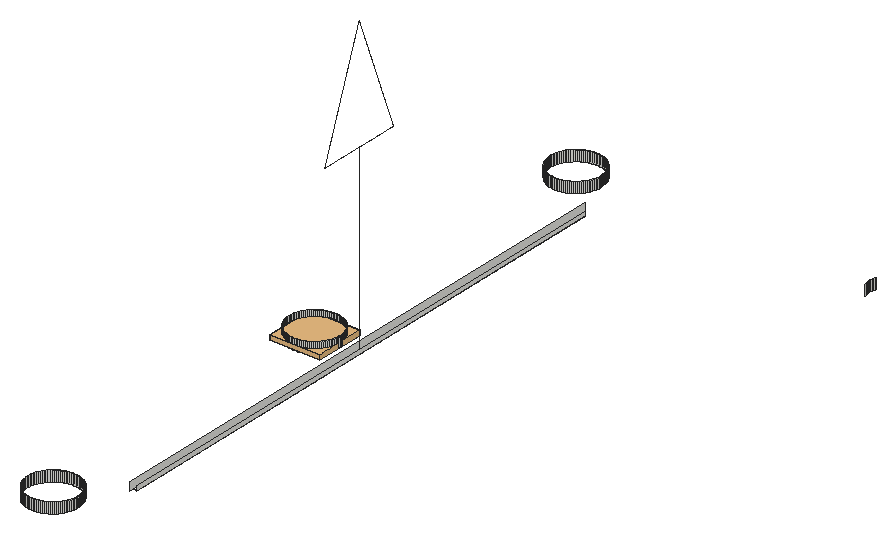
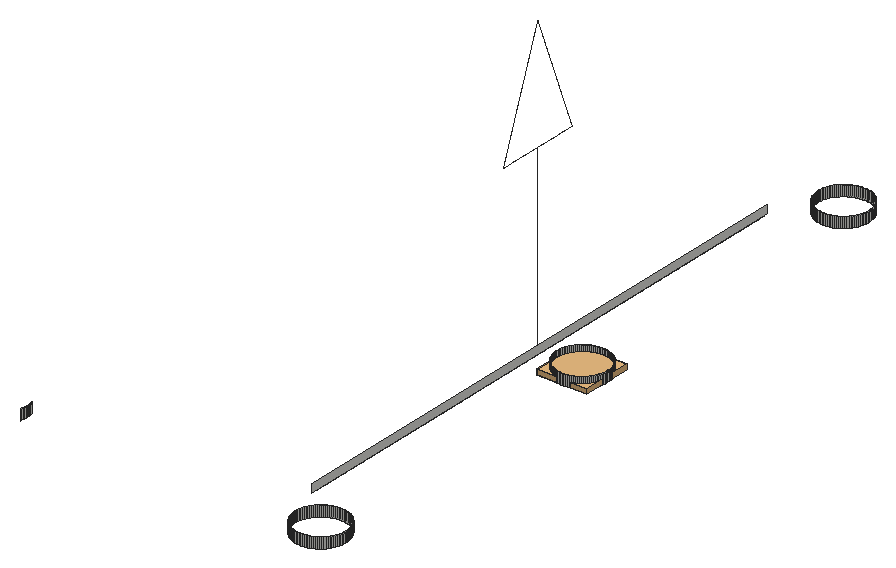
# SketchUp Ruby script. Lengths in inches.
U = 1.inch
M = Sketchup.active_model
def pt(a) = Geom::Point3d.new(a.map { |v| v * U })
def face(e, loops, mat)
  f = e.add_face(loops[0].map { |a| pt(a) })
  loops[1..].each { |l| e.add_face(l.map { |a| pt(a) }).erase! }
  f.material = f.back_material = mat if mat
  f
end
# faces: each face lists its corners as indices into pts; further lists are holes
def faces(e, pts, list, mat = nil) = list.each { |f| face(e, (f[0].is_a?(Array) ? f : [f]).map { |l| l.map { |i| pts[i] } }, mat) }
# xy, xz, yz: faces in a plane at the given z, y or x. An outline is a flat list of corners, or four numbers for a rectangle; further outlines are holes
def ring(l) = l.size == 4 ? [[l[0], l[1]], [l[2], l[1]], [l[2], l[3]], [l[0], l[3]]] : l.each_slice(2).to_a
def flat(e, list, mat, &to3) = list.each { |f| face(e, (f[0].is_a?(Array) ? f : [f]).map { |l| ring(l).map { |u, v| to3.(u, v) } }, mat) }
def xy(e, z, list, mat = nil) = flat(e, list, mat) { |x, y| [x, y, z] }
def xz(e, y, list, mat = nil) = flat(e, list, mat) { |x, z| [x, y, z] }
def yz(e, x, list, mat = nil) = flat(e, list, mat) { |y, z| [x, y, z] }
def lines(e, pts, list) = list.each { |a, b| e.add_line(pt(pts[a]), pt(pts[b])) }
# prism: a flat outline (further loops are holes) pulled along v
def prism(e, loops, v, mat = nil)
  f = face(e, loops, mat); d = Geom::Vector3d.new(v.map { |x| x * U })
  f.pushpull(f.normal.samedirection?(d) ? d.length : -d.length)
end
def box(e, o, s, mat = nil) = prism(e, [[o, [o[0] + s[0], o[1], o[2]], [o[0] + s[0], o[1] + s[1], o[2]], [o[0], o[1] + s[1], o[2]]]], [0, 0, s[2]], mat)
def at(x, y, z, deg = 0) = Geom::Transformation.translation(pt([x, y, z])) * Geom::Transformation.rotation(ORIGIN, Z_AXIS, deg.degrees)
def axes(o, x, y, z) = Geom::Transformation.new([*x, 0, *y, 0, *z, 0, *pt(o).to_a, 1])
def part(name) = M.definitions.add(name)
# library, detail: a bought-in or finely detailed component or shape, given as its bounding box
def library(name, o, s) = part(name).tap { |d| box(d.entities, o, s) }
def detail(e, o, s) = box(e.add_group.entities, o, s)
def put(e, d, t, mat = nil) = e.add_instance(d, t).tap { |i| i.material = mat if mat }
def group(e, t, mat = nil) = e.add_group.tap { |g| g.transformation = t; g.material = mat if mat }.entities
root = M.entities
c1 = library("plafonjera p5",[102.27,51.27,12.6],[3.93,3.93,0.39])
c2 = part("Group84\#1")
p = [[0,0,0],[0,0,-43.36],[-21.49,0,-43.36],[139.88,-0.5,0],[-139.88,-0.5,0],[139.88,0.5,0],
  [139.88,0,0],[-139.88,0.5,0],[21.49,0,-43.36],[-139.88,0,0],[0,0,-70.19]]
lines(c2.entities,p,[[0,1],[1,2],[3,4],[5,6],[7,5],[1,8],[9,0],[0,6],[8,10],[4,9],[6,3],[2,10],
  [9,7]])
c3 = part("Rectangle Light")
put(c3.entities,c2,at(0,0,0))
xy(root,231.53,[[64.14,38.69,64.07,39.0625,64.02,39.44]])
xz(root,34,[[69.8,231.53,70.18,234]])
xz(root,46,[[69.8,231.53,70.18,234]])
xz(root,111,[[69.8,231.53,70.18,234]])
xz(root,123,[[69.8,231.53,70.18,234]])
xz(root,188,[[69.8,231.53,70.18,234]])
xz(root,200,[[69.8,231.53,70.18,234]])
yz(root,63.99,[[39.8125,231.53,40.1875,234],[116.8125,231.53,117.1875,234],[193.8125,231.53,194.1875,234]])
yz(root,75.99,[[39.8125,231.53,40.1875,234],[116.8125,231.53,117.1875,234],[193.8125,231.53,194.1875,234]])
yz(root,79.99,[[50,232,184,234]])
yz(root,80.99,[[51,232,183,233]])
yz(root,139.18,[[193.8125,231.53,194.1875,234]])
p = [[69.43,34.03,231.53],[69.05,34.07,231.53],[69.05,34.07,234],[69.43,34.03,234],[69.8,34,231.53],[69.8,34,234],
  [70.56,34.03,231.53],[70.18,34,231.53],[70.18,34,234],[70.56,34.03,234],[70.93,34.07,231.53],[70.93,34.07,234],
  [68.68,34.14,231.53],[68.32,34.24,231.53],[68.32,34.24,234],[68.68,34.14,234],[71.3,34.14,231.53],[71.3,34.14,234],
  [71.67,34.24,231.53],[71.67,34.24,234],[67.96,34.35,231.53],[67.96,34.35,234],[72.02,34.35,231.53],[72.02,34.35,234],
  [67.61,34.49,231.53],[67.61,34.49,234],[72.375,34.49,231.53],[72.375,34.49,234],[67.27,34.65,231.53],[67.27,34.65,234],
  [72.72,34.65,231.53],[72.72,34.65,234],[66.9375,34.84,231.53],[66.9375,34.84,234],[73.05,34.84,231.53],[73.05,34.84,234],
  [66.62,35.04,231.53],[66.62,35.04,234],[73.36,35.04,231.53],[73.36,35.04,234],[66.3125,35.26,231.53],[66.3125,35.26,234],
  [73.67,35.26,231.53],[73.67,35.26,234],[66.02,35.5,231.53],[66.02,35.5,234],[73.96,35.5,231.53],[73.96,35.5,234],
  [65.75,35.76,231.53],[65.75,35.76,234],[74.23,35.76,231.53],[74.23,35.76,234],[65.49,36.03,231.53],[65.49,36.03,234],
  [74.49,36.03,231.53],[74.49,36.03,234],[65.25,36.32,231.53],[65.25,36.32,234],[74.73,36.32,231.53],[74.73,36.32,234],
  [65.03,36.63,231.53],[65.03,36.63,234],[74.95,36.63,231.53],[74.95,36.63,234],[64.83,36.95,231.53],[64.83,36.95,234],
  [75.16,36.95,231.53],[75.16,36.95,234],[64.65,37.28,231.53],[64.65,37.28,234],[75.34,37.28,231.53],[75.34,37.28,234],
  [64.48,37.62,231.53],[64.48,37.62,234],[75.5,37.62,231.53],[75.5,37.62,234],[64.35,37.97,231.53],[64.35,37.97,234],
  [75.64,37.97,231.53],[75.64,37.97,234],[64.23,38.33,231.53],[64.23,38.33,234],[75.75,38.33,231.53],[75.75,38.33,234],
  [64.14,38.69,231.53],[64.14,38.69,234],[75.85,38.69,231.53],[75.85,38.69,234],[75.92,39.0625,231.53],[75.92,39.0625,234],
  [75.96,39.44,231.53],[75.96,39.44,234],[64.02,39.44,231.53],[63.99,39.8125,231.53],[63.99,39.8125,234],[64.02,39.44,234],
  [75.99,39.8125,231.53],[75.99,39.8125,234],[63.99,40.1875,231.53],[64.02,40.56,231.53],[64.02,40.56,234],[63.99,40.1875,234],
  [75.96,40.56,231.53],[75.99,40.1875,231.53],[75.99,40.1875,234],[75.96,40.56,234],[64.07,40.9375,231.53],[64.07,40.9375,234],
  [75.92,40.9375,231.53],[75.92,40.9375,234],[64.14,41.31,231.53],[64.14,41.31,234],[75.85,41.31,231.53],[75.85,41.31,234],
  [64.23,41.67,231.53],[64.23,41.67,234],[75.75,41.67,231.53],[75.75,41.67,234],[64.35,42.03,231.53],[64.35,42.03,234],
  [75.64,42.03,231.53],[75.64,42.03,234],[64.48,42.38,231.53],[64.48,42.38,234],[75.5,42.38,231.53],[75.5,42.38,234],
  [64.65,42.72,231.53],[64.65,42.72,234],[75.34,42.72,231.53],[75.34,42.72,234],[64.83,43.05,231.53],[64.83,43.05,234],
  [75.16,43.05,231.53],[75.16,43.05,234],[65.03,43.37,231.53],[65.03,43.37,234],[74.95,43.37,231.53],[74.95,43.37,234],
  [65.25,43.68,231.53],[65.25,43.68,234],[74.73,43.68,231.53],[74.73,43.68,234],[65.49,43.97,231.53],[65.49,43.97,234],
  [74.49,43.97,231.53],[74.49,43.97,234],[65.75,44.24,231.53],[65.75,44.24,234],[74.23,44.24,231.53],[74.23,44.24,234],
  [66.02,44.5,231.53],[66.02,44.5,234],[73.96,44.5,231.53],[73.96,44.5,234],[66.3125,44.74,231.53],[66.3125,44.74,234],
  [73.67,44.74,231.53],[73.67,44.74,234],[66.62,44.96,231.53],[66.62,44.96,234],[73.36,44.96,231.53],[73.36,44.96,234],
  [66.9375,45.16,231.53],[66.9375,45.16,234],[73.05,45.16,231.53],[73.05,45.16,234],[67.27,45.35,231.53],[67.27,45.35,234],
  [72.72,45.35,231.53],[72.72,45.35,234],[67.61,45.51,231.53],[67.61,45.51,234],[72.375,45.51,231.53],[72.375,45.51,234],
  [67.96,45.65,231.53],[67.96,45.65,234],[72.02,45.65,231.53],[72.02,45.65,234],[68.32,45.76,231.53],[68.32,45.76,234],
  [71.67,45.76,231.53],[71.67,45.76,234],[68.68,45.86,231.53],[68.68,45.86,234],[71.3,45.86,231.53],[71.3,45.86,234],
  [69.05,45.93,231.53],[69.05,45.93,234],[69.43,45.97,231.53],[69.43,45.97,234],[70.56,45.97,231.53],[70.93,45.93,231.53],
  [70.93,45.93,234],[70.56,45.97,234],[69.8,46,231.53],[69.8,46,234],[70.18,46,231.53],[70.18,46,234],
  [69.43,111.03,231.53],[69.05,111.07,231.53],[69.05,111.07,234],[69.43,111.03,234],[69.8,111,231.53],[69.8,111,234],
  [70.56,111.03,231.53],[70.18,111,231.53],[70.18,111,234],[70.56,111.03,234],[70.93,111.07,231.53],[70.93,111.07,234],
  [68.68,111.14,231.53],[68.32,111.24,231.53],[68.32,111.24,234],[68.68,111.14,234],[71.3,111.14,231.53],[71.3,111.14,234],
  [71.67,111.24,231.53],[71.67,111.24,234],[67.96,111.35,231.53],[67.96,111.35,234],[72.02,111.35,231.53],[72.02,111.35,234],
  [67.61,111.49,231.53],[67.61,111.49,234],[72.375,111.49,231.53],[72.375,111.49,234],[67.27,111.65,231.53],[67.27,111.65,234],
  [72.72,111.65,231.53],[72.72,111.65,234],[66.9375,111.84,231.53],[66.9375,111.84,234],[73.05,111.84,231.53],[73.05,111.84,234],
  [66.62,112.04,231.53],[66.62,112.04,234],[73.36,112.04,231.53],[73.36,112.04,234],[66.3125,112.26,231.53],[66.3125,112.26,234],
  [73.67,112.26,231.53],[73.67,112.26,234],[66.02,112.5,231.53],[66.02,112.5,234],[73.96,112.5,231.53],[73.96,112.5,234],
  [65.75,112.76,231.53],[65.75,112.76,234],[74.23,112.76,231.53],[74.23,112.76,234],[65.49,113.03,231.53],[65.49,113.03,234],
  [74.49,113.03,231.53],[74.49,113.03,234],[65.25,113.32,231.53],[65.25,113.32,234],[74.73,113.32,231.53],[74.73,113.32,234],
  [65.03,113.63,231.53],[65.03,113.63,234],[74.95,113.63,231.53],[74.95,113.63,234],[64.83,113.95,231.53],[64.83,113.95,234],
  [75.16,113.95,231.53],[75.16,113.95,234],[64.65,114.28,231.53],[64.65,114.28,234],[75.34,114.28,231.53],[75.34,114.28,234],
  [64.48,114.62,231.53],[64.48,114.62,234],[75.5,114.62,231.53],[75.5,114.62,234],[64.35,114.97,231.53],[64.35,114.97,234],
  [75.64,114.97,231.53],[75.64,114.97,234],[64.23,115.33,231.53],[64.23,115.33,234],[75.75,115.33,231.53],[75.75,115.33,234],
  [64.14,115.69,231.53],[64.14,115.69,234],[75.85,115.69,231.53],[75.85,115.69,234],[64.07,116.0625,231.53],[64.07,116.0625,234],
  [75.92,116.0625,231.53],[75.92,116.0625,234],[64.02,116.44,231.53],[64.02,116.44,234],[75.96,116.44,231.53],[75.96,116.44,234],
  [63.99,116.8125,231.53],[63.99,116.8125,234],[75.99,116.8125,231.53],[75.99,116.8125,234],[63.99,117.1875,231.53],[64.02,117.56,231.53],
  [64.02,117.56,234],[63.99,117.1875,234],[75.96,117.56,231.53],[75.99,117.1875,231.53],[75.99,117.1875,234],[75.96,117.56,234],
  [64.07,117.9375,231.53],[64.07,117.9375,234],[75.92,117.9375,231.53],[75.92,117.9375,234],[64.14,118.31,231.53],[64.14,118.31,234],
  [75.85,118.31,231.53],[75.85,118.31,234],[64.23,118.67,231.53],[64.23,118.67,234],[75.75,118.67,231.53],[75.75,118.67,234],
  [64.35,119.03,231.53],[64.35,119.03,234],[75.64,119.03,231.53],[75.64,119.03,234],[64.48,119.38,231.53],[64.48,119.38,234],
  [75.5,119.38,231.53],[75.5,119.38,234],[64.65,119.72,231.53],[64.65,119.72,234],[75.34,119.72,231.53],[75.34,119.72,234],
  [64.83,120.05,231.53],[64.83,120.05,234],[75.16,120.05,231.53],[75.16,120.05,234],[65.03,120.37,231.53],[65.03,120.37,234],
  [74.95,120.37,231.53],[74.95,120.37,234],[65.25,120.68,231.53],[65.25,120.68,234],[74.73,120.68,231.53],[74.73,120.68,234],
  [65.49,120.97,231.53],[65.49,120.97,234],[74.49,120.97,231.53],[74.49,120.97,234],[65.75,121.24,231.53],[65.75,121.24,234],
  [74.23,121.24,231.53],[74.23,121.24,234],[66.02,121.5,231.53],[66.02,121.5,234],[73.96,121.5,231.53],[73.96,121.5,234],
  [66.3125,121.74,231.53],[66.3125,121.74,234],[73.67,121.74,231.53],[73.67,121.74,234],[66.62,121.96,231.53],[66.62,121.96,234],
  [73.36,121.96,231.53],[73.36,121.96,234],[66.9375,122.16,231.53],[66.9375,122.16,234],[73.05,122.16,231.53],[73.05,122.16,234],
  [67.27,122.35,231.53],[67.27,122.35,234],[72.72,122.35,231.53],[72.72,122.35,234],[67.61,122.51,231.53],[67.61,122.51,234],
  [72.375,122.51,231.53],[72.375,122.51,234],[67.96,122.65,231.53],[67.96,122.65,234],[72.02,122.65,231.53],[72.02,122.65,234],
  [68.32,122.76,231.53],[68.32,122.76,234],[71.67,122.76,231.53],[71.67,122.76,234],[68.68,122.86,231.53],[68.68,122.86,234],
  [71.3,122.86,231.53],[71.3,122.86,234],[69.05,122.93,231.53],[69.05,122.93,234],[69.43,122.97,231.53],[69.43,122.97,234],
  [70.56,122.97,231.53],[70.93,122.93,231.53],[70.93,122.93,234],[70.56,122.97,234],[69.8,123,231.53],[69.8,123,234],
  [70.18,123,231.53],[70.18,123,234],[69.43,188.03,231.53],[69.05,188.07,231.53],[69.05,188.07,234],[69.43,188.03,234],
  [69.8,188,231.53],[69.8,188,234],[70.56,188.03,231.53],[70.18,188,231.53],[70.18,188,234],[70.56,188.03,234],
  [70.93,188.07,231.53],[70.93,188.07,234],[68.68,188.14,231.53],[68.32,188.24,231.53],[68.32,188.24,234],[68.68,188.14,234],
  [71.3,188.14,231.53],[71.3,188.14,234],[71.67,188.24,231.53],[71.67,188.24,234],[67.96,188.35,231.53],[67.96,188.35,234],
  [72.02,188.35,231.53],[72.02,188.35,234],[67.61,188.49,231.53],[67.61,188.49,234],[72.375,188.49,231.53],[72.375,188.49,234],
  [67.27,188.65,231.53],[67.27,188.65,234],[72.72,188.65,231.53],[72.72,188.65,234],[66.9375,188.84,231.53],[66.9375,188.84,234],
  [73.05,188.84,231.53],[73.05,188.84,234],[66.62,189.04,231.53],[66.62,189.04,234],[73.36,189.04,231.53],[73.36,189.04,234],
  [66.3125,189.26,231.53],[66.3125,189.26,234],[73.67,189.26,231.53],[73.67,189.26,234],[66.02,189.5,231.53],[66.02,189.5,234],
  [73.96,189.5,231.53],[73.96,189.5,234],[65.75,189.76,231.53],[65.75,189.76,234],[74.23,189.76,231.53],[74.23,189.76,234],
  [65.49,190.03,231.53],[65.49,190.03,234],[74.49,190.03,231.53],[74.49,190.03,234],[65.25,190.32,231.53],[65.25,190.32,234],
  [74.73,190.32,231.53],[74.73,190.32,234],[65.03,190.63,231.53],[65.03,190.63,234],[74.95,190.63,231.53],[74.95,190.63,234],
  [64.83,190.95,231.53],[64.83,190.95,234],[75.16,190.95,231.53],[75.16,190.95,234],[64.65,191.28,231.53],[64.65,191.28,234],
  [75.34,191.28,231.53],[75.34,191.28,234],[64.48,191.62,231.53],[64.48,191.62,234],[75.5,191.62,231.53],[75.5,191.62,234],
  [64.35,191.97,231.53],[64.35,191.97,234],[75.64,191.97,231.53],[75.64,191.97,234],[64.23,192.33,231.53],[64.23,192.33,234],
  [75.75,192.33,231.53],[75.75,192.33,234],[64.14,192.69,231.53],[64.14,192.69,234],[75.85,192.69,231.53],[75.85,192.69,234],
  [139.42,192.33,231.53],[139.33,192.69,231.53],[139.33,192.69,234],[139.42,192.33,234],[64.07,193.0625,231.53],[64.07,193.0625,234],
  [75.92,193.0625,231.53],[75.92,193.0625,234],[139.26,193.0625,231.53],[139.26,193.0625,234],[64.02,193.44,231.53],[64.02,193.44,234],
  [75.96,193.44,231.53],[75.96,193.44,234],[139.21,193.44,231.53],[139.21,193.44,234],[63.99,193.8125,231.53],[63.99,193.8125,234],
  [75.99,193.8125,231.53],[75.99,193.8125,234],[139.18,193.8125,231.53],[139.18,193.8125,234],[63.99,194.1875,231.53],[64.02,194.56,231.53],
  [64.02,194.56,234],[63.99,194.1875,234],[75.96,194.56,231.53],[75.99,194.1875,231.53],[75.99,194.1875,234],[75.96,194.56,234],
  [139.18,194.1875,231.53],[139.21,194.56,231.53],[139.21,194.56,234],[139.18,194.1875,234],[64.07,194.9375,231.53],[64.07,194.9375,234],
  [75.92,194.9375,231.53],[75.92,194.9375,234],[139.26,194.9375,231.53],[139.26,194.9375,234],[64.14,195.31,231.53],[64.14,195.31,234],
  [75.85,195.31,231.53],[75.85,195.31,234],[139.33,195.31,231.53],[139.33,195.31,234],[64.23,195.67,231.53],[64.23,195.67,234],
  [75.75,195.67,231.53],[75.75,195.67,234],[139.42,195.67,231.53],[139.42,195.67,234],[64.35,196.03,231.53],[64.35,196.03,234],
  [75.64,196.03,231.53],[75.64,196.03,234],[64.48,196.38,231.53],[64.48,196.38,234],[75.5,196.38,231.53],[75.5,196.38,234],
  [64.65,196.72,231.53],[64.65,196.72,234],[75.34,196.72,231.53],[75.34,196.72,234],[64.83,197.05,231.53],[64.83,197.05,234],
  [75.16,197.05,231.53],[75.16,197.05,234],[65.03,197.37,231.53],[65.03,197.37,234],[74.95,197.37,231.53],[74.95,197.37,234],
  [65.25,197.68,231.53],[65.25,197.68,234],[74.73,197.68,231.53],[74.73,197.68,234],[65.49,197.97,231.53],[65.49,197.97,234],
  [74.49,197.97,231.53],[74.49,197.97,234],[65.75,198.24,231.53],[65.75,198.24,234],[74.23,198.24,231.53],[74.23,198.24,234],
  [66.02,198.5,231.53],[66.02,198.5,234],[73.96,198.5,231.53],[73.96,198.5,234],[66.3125,198.74,231.53],[66.3125,198.74,234],
  [73.67,198.74,231.53],[73.67,198.74,234],[66.62,198.96,231.53],[66.62,198.96,234],[73.36,198.96,231.53],[73.36,198.96,234],
  [66.9375,199.16,231.53],[66.9375,199.16,234],[73.05,199.16,231.53],[73.05,199.16,234],[67.27,199.35,231.53],[67.27,199.35,234],
  [72.72,199.35,231.53],[72.72,199.35,234],[67.61,199.51,231.53],[67.61,199.51,234],[72.375,199.51,231.53],[72.375,199.51,234],
  [67.96,199.65,231.53],[67.96,199.65,234],[72.02,199.65,231.53],[72.02,199.65,234],[68.32,199.76,231.53],[68.32,199.76,234],
  [71.67,199.76,231.53],[71.67,199.76,234],[68.68,199.86,231.53],[68.68,199.86,234],[71.3,199.86,231.53],[71.3,199.86,234],
  [69.05,199.93,231.53],[69.05,199.93,234],[69.43,199.97,231.53],[69.43,199.97,234],[70.56,199.97,231.53],[70.93,199.93,231.53],
  [70.93,199.93,234],[70.56,199.97,234],[69.8,200,231.53],[69.8,200,234],[70.18,200,231.53],[70.18,200,234]]
faces(root,p,[[0,1,2,3],[4,0,3,5],[6,7,8,9],[10,6,9,11],[12,13,14,15],[1,12,15,2],[16,10,11,17],[18,16,17,19],
  [13,20,21,14],[22,18,19,23],[20,24,25,21],[26,22,23,27],[24,28,29,25],[30,26,27,31],[28,32,33,29],[34,30,31,35],
  [32,36,37,33],[38,34,35,39],[36,40,41,37],[42,38,39,43],[40,44,45,41],[46,42,43,47],[44,48,49,45],[50,46,47,51],
  [48,52,53,49],[54,50,51,55],[52,56,57,53],[58,54,55,59],[56,60,61,57],[62,58,59,63],[60,64,65,61],[66,62,63,67],
  [64,68,69,65],[70,66,67,71],[68,72,73,69],[74,70,71,75],[72,76,77,73],[78,74,75,79],[76,80,81,77],[82,78,79,83],
  [80,84,85,81],[86,82,83,87],[88,86,87,89],[90,88,89,91],[92,93,94,95],[96,90,91,97],[98,99,100,101],[102,103,104,105],
  [99,106,107,100],[108,102,105,109],[106,110,111,107],[112,108,109,113],[110,114,115,111],[116,112,113,117],[114,118,119,115],[120,116,117,121],
  [118,122,123,119],[124,120,121,125],[122,126,127,123],[128,124,125,129],[126,130,131,127],[132,128,129,133],[130,134,135,131],[136,132,133,137],
  [134,138,139,135],[140,136,137,141],[138,142,143,139],[144,140,141,145],[142,146,147,143],[148,144,145,149],[146,150,151,147],[152,148,149,153],
  [150,154,155,151],[156,152,153,157],[154,158,159,155],[160,156,157,161],[158,162,163,159],[164,160,161,165],[162,166,167,163],[168,164,165,169],
  [166,170,171,167],[172,168,169,173],[170,174,175,171],[176,172,173,177],[174,178,179,175],[180,176,177,181],[178,182,183,179],[184,180,181,185],
  [182,186,187,183],[186,188,189,187],[190,191,192,193],[191,184,185,192],[188,194,195,189],[196,190,193,197],[198,199,200,201],[202,198,201,203],
  [204,205,206,207],[208,204,207,209],[210,211,212,213],[199,210,213,200],[214,208,209,215],[216,214,215,217],[211,218,219,212],[220,216,217,221],
  [218,222,223,219],[224,220,221,225],[222,226,227,223],[228,224,225,229],[226,230,231,227],[232,228,229,233],[230,234,235,231],[236,232,233,237],
  [234,238,239,235],[240,236,237,241],[238,242,243,239],[244,240,241,245],[242,246,247,243],[248,244,245,249],[246,250,251,247],[252,248,249,253],
  [250,254,255,251],[256,252,253,257],[254,258,259,255],[260,256,257,261],[258,262,263,259],[264,260,261,265],[262,266,267,263],[268,264,265,269],
  [266,270,271,267],[272,268,269,273],[270,274,275,271],[276,272,273,277],[274,278,279,275],[280,276,277,281],[278,282,283,279],[284,280,281,285],
  [282,286,287,283],[288,284,285,289],[286,290,291,287],[292,288,289,293],[290,294,295,291],[296,292,293,297],[298,299,300,301],[302,303,304,305],
  [299,306,307,300],[308,302,305,309],[306,310,311,307],[312,308,309,313],[310,314,315,311],[316,312,313,317],[314,318,319,315],[320,316,317,321],
  [318,322,323,319],[324,320,321,325],[322,326,327,323],[328,324,325,329],[326,330,331,327],[332,328,329,333],[330,334,335,331],[336,332,333,337],
  [334,338,339,335],[340,336,337,341],[338,342,343,339],[344,340,341,345],[342,346,347,343],[348,344,345,349],[346,350,351,347],[352,348,349,353],
  [350,354,355,351],[356,352,353,357],[354,358,359,355],[360,356,357,361],[358,362,363,359],[364,360,361,365],[362,366,367,363],[368,364,365,369],
  [366,370,371,367],[372,368,369,373],[370,374,375,371],[376,372,373,377],[374,378,379,375],[380,376,377,381],[378,382,383,379],[384,380,381,385],
  [382,386,387,383],[386,388,389,387],[390,391,392,393],[391,384,385,392],[388,394,395,389],[396,390,393,397],[398,399,400,401],[402,398,401,403],
  [404,405,406,407],[408,404,407,409],[410,411,412,413],[399,410,413,400],[414,408,409,415],[416,414,415,417],[411,418,419,412],[420,416,417,421],
  [418,422,423,419],[424,420,421,425],[422,426,427,423],[428,424,425,429],[426,430,431,427],[432,428,429,433],[430,434,435,431],[436,432,433,437],
  [434,438,439,435],[440,436,437,441],[438,442,443,439],[444,440,441,445],[442,446,447,443],[448,444,445,449],[446,450,451,447],[452,448,449,453],
  [450,454,455,451],[456,452,453,457],[454,458,459,455],[460,456,457,461],[458,462,463,459],[464,460,461,465],[462,466,467,463],[468,464,465,469],
  [466,470,471,467],[472,468,469,473],[470,474,475,471],[476,472,473,477],[474,478,479,475],[480,476,477,481],[478,482,483,479],[484,480,481,485],
  [486,487,488,489],[482,490,491,483],[492,484,485,493],[487,494,495,488],[490,496,497,491],[498,492,493,499],[494,500,501,495],[496,502,503,497],
  [504,498,499,505],[500,506,507,501],[508,509,510,511],[512,513,514,515],[516,517,518,519],[509,520,521,510],[522,512,515,523],[517,524,525,518],
  [520,526,527,521],[528,522,523,529],[524,530,531,525],[526,532,533,527],[534,528,529,535],[530,536,537,531],[532,538,539,533],[540,534,535,541],
  [538,542,543,539],[544,540,541,545],[542,546,547,543],[548,544,545,549],[546,550,551,547],[552,548,549,553],[550,554,555,551],[556,552,553,557],
  [554,558,559,555],[560,556,557,561],[558,562,563,559],[564,560,561,565],[562,566,567,563],[568,564,565,569],[566,570,571,567],[572,568,569,573],
  [570,574,575,571],[576,572,573,577],[574,578,579,575],[580,576,577,581],[578,582,583,579],[584,580,581,585],[582,586,587,583],[588,584,585,589],
  [586,590,591,587],[592,588,589,593],[590,594,595,591],[596,592,593,597],[594,598,599,595],[600,596,597,601],[598,602,603,599],[604,600,601,605],
  [602,606,607,603],[606,608,609,607],[610,611,612,613],[611,604,605,612],[608,614,615,609],[616,610,613,617]])
put(root,c1,axes([-242.63,-42.83,193.73],[3,0,0],[0,3,0],[0,0,3]))
put(root,c3,axes([80.49,117,232.01],[0,-0.47184,0],[-1,0,0],[0,0,-1]))
